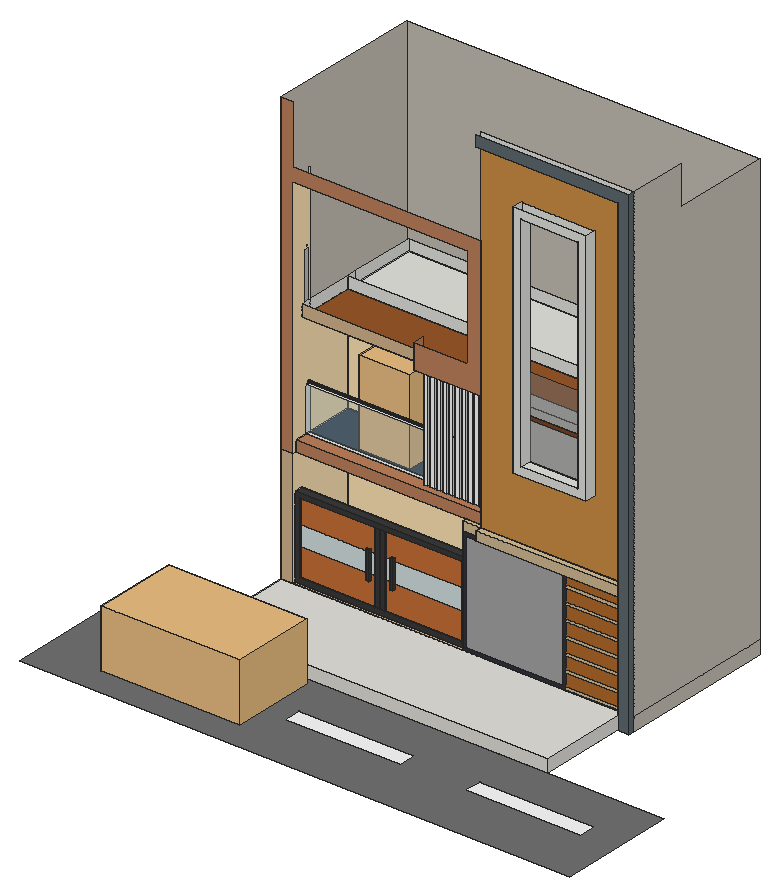
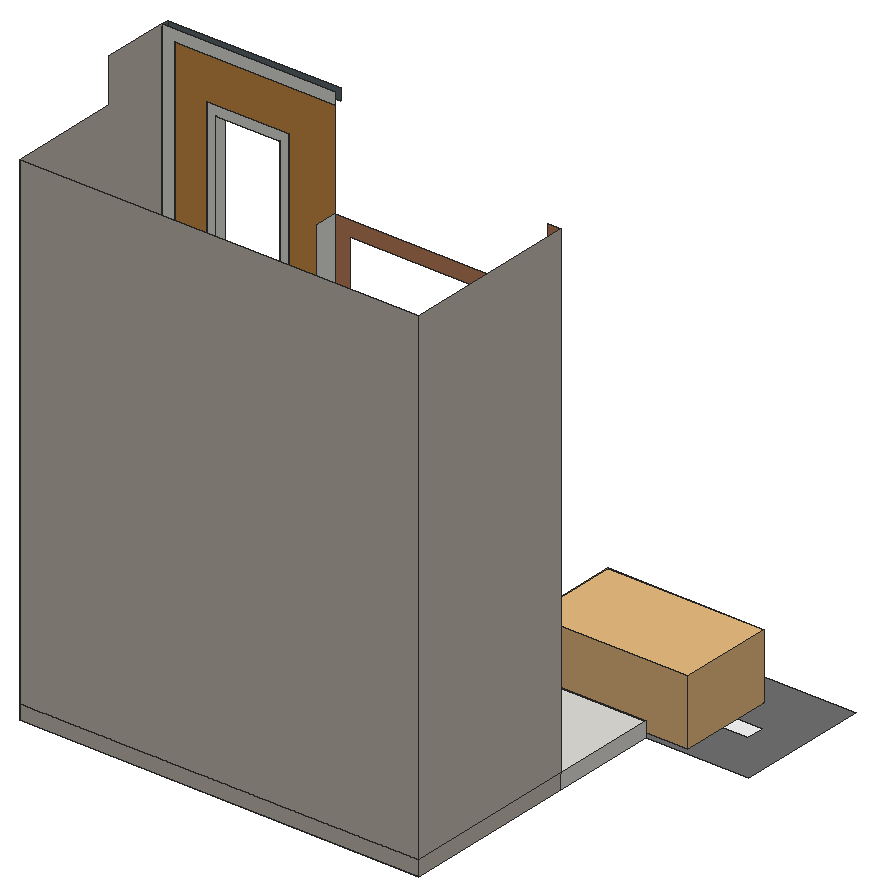
# SketchUp Ruby script. Lengths in inches.
U = 1.inch
M = Sketchup.active_model
def pt(a) = Geom::Point3d.new(a.map { |v| v * U })
def face(e, loops, mat)
  f = e.add_face(loops[0].map { |a| pt(a) })
  loops[1..].each { |l| e.add_face(l.map { |a| pt(a) }).erase! }
  f.material = f.back_material = mat if mat
  f
end
# faces: each face lists its corners as indices into pts; further lists are holes
def faces(e, pts, list, mat = nil) = list.each { |f| face(e, (f[0].is_a?(Array) ? f : [f]).map { |l| l.map { |i| pts[i] } }, mat) }
# xy, xz, yz: faces in a plane at the given z, y or x. An outline is a flat list of corners, or four numbers for a rectangle; further outlines are holes
def ring(l) = l.size == 4 ? [[l[0], l[1]], [l[2], l[1]], [l[2], l[3]], [l[0], l[3]]] : l.each_slice(2).to_a
def flat(e, list, mat, &to3) = list.each { |f| face(e, (f[0].is_a?(Array) ? f : [f]).map { |l| ring(l).map { |u, v| to3.(u, v) } }, mat) }
def xy(e, z, list, mat = nil) = flat(e, list, mat) { |x, y| [x, y, z] }
def xz(e, y, list, mat = nil) = flat(e, list, mat) { |x, z| [x, y, z] }
def yz(e, x, list, mat = nil) = flat(e, list, mat) { |y, z| [x, y, z] }
def lines(e, pts, list) = list.each { |a, b| e.add_line(pt(pts[a]), pt(pts[b])) }
# prism: a flat outline (further loops are holes) pulled along v
def prism(e, loops, v, mat = nil)
  f = face(e, loops, mat); d = Geom::Vector3d.new(v.map { |x| x * U })
  f.pushpull(f.normal.samedirection?(d) ? d.length : -d.length)
end
def box(e, o, s, mat = nil) = prism(e, [[o, [o[0] + s[0], o[1], o[2]], [o[0] + s[0], o[1] + s[1], o[2]], [o[0], o[1] + s[1], o[2]]]], [0, 0, s[2]], mat)
def at(x, y, z, deg = 0) = Geom::Transformation.translation(pt([x, y, z])) * Geom::Transformation.rotation(ORIGIN, Z_AXIS, deg.degrees)
def axes(o, x, y, z) = Geom::Transformation.new([*x, 0, *y, 0, *z, 0, *pt(o).to_a, 1])
def part(name) = M.definitions.add(name)
# library, detail: a bought-in or finely detailed component or shape, given as its bounding box
def library(name, o, s) = part(name).tap { |d| box(d.entities, o, s) }
def detail(e, o, s) = box(e.add_group.entities, o, s)
def put(e, d, t, mat = nil) = e.add_instance(d, t).tap { |i| i.material = mat if mat }
def group(e, t, mat = nil) = e.add_group.tap { |g| g.transformation = t; g.material = mat if mat }.entities
root = M.entities
M.materials.add("[0032_Moccasin]").color = [255, 228, 181]
M.materials.add("[0035_Tan]").color = [210, 180, 140]
M.materials.add("[Carpet Pattern Leaf Squares Tan]").color = [181, 154, 125]
M.materials.add("[Color M05]").color = [114, 114, 114]
M.materials.add("[Color M07]").color = [58, 58, 58]
M.materials.add("[Field Rectangle Tile]").color = [196, 189, 179]
M.materials.add("[Formica Beige]").color = [211, 187, 149]
M.materials.add("[Formica Laminate Dark]").color = [50, 53, 60]
M.materials.add("[Formica Speckled Grey]").color = [94, 105, 111]
M.materials.add("[Leather Blue]").color = [45, 57, 74]
M.materials.add("[Marble Carrara Gold Floor Tile]").color = [225, 223, 217]
M.materials.add("[Quartz Light Grey]").color = [251, 251, 252]
M.materials.add("[Stone Vein Gray]").color = [166, 165, 165]
M.materials.add("[Translucent Glass Gray]").color = [128, 128, 128]
M.materials["[Translucent Glass Gray]"].alpha = 0.5
M.materials.add("[Translucent Glass Safety]").color = [204, 235, 244]
M.materials["[Translucent Glass Safety]"].alpha = 0.14
M.materials.add("[Wallpaper Dog Bone]").color = [213, 224, 224]
M.materials.add("[Wallpaper Stripe]").color = [204, 141, 68]
M.materials.add("[Wood Bamboo]").color = [177, 105, 43]
M.materials.add("[Wood Cherry Original]").color = [198, 112, 54]
M.materials.add("[Wood Cherry Original]1").color = [152, 86, 42]
M.materials.add("[Wood Veneer 01]").color = [120, 70, 37]
M.materials.add("[Wood Veneer 02]").color = [190, 128, 91]
c1 = library("skpE847",[-111.76,-15.01,0.76],[2.12,4.6,1.82])
c2 = part("car+1")
p = [[0,0,0],[1,0,0],[1,1,0]]
lines(c2.entities,p,[[0,1],[1,2],[2,0]])
put(c2.entities,c1,axes([-477.97,5140.8,-31.25],[0,46,0],[-46,0,0],[0,0,40.94]))
c3 = library("chau cay",[-24.34,-109.24,0],[56.46,62.58,79.69])
xy(root,0,[[663.13,313.84,680.56,323.28],[140.56,323.28,680.56,563.28]])
xy(root,0,[[[0,0,841.5625,179.6875],[54.75,86.11,232.01,113.17],[336.5,86.11,513.76,113.17],[612.25,86.11,789.51,113.17]]],"[Color M05]")
xy(root,0,[[140.56,179.6875,663.13,323.28]],"[Marble Carrara Gold Floor Tile]")
xy(root,0,[[54.75,86.11,232.01,113.17],[336.5,86.11,513.76,113.17],[612.25,86.11,789.51,113.17]],"[Quartz Light Grey]")
xy(root,19.8125,[[419.17,323.28,663.13,340.7],[663.13,323.28,680.56,428.92],[157.98,328.46,419.17,340.7],[157.98,428.92,663.13,443.28],[157.98,443.28,663.13,545.86]])
xy(root,19.8125,[[157.98,323.28,419.17,328.46]],"[0035_Tan]")
xy(root,19.8125,[[157.98,340.7,663.13,428.92]],"[Carpet Pattern Leaf Squares Tan]")
xy(root,19.8125,[[140.56,179.6875,663.13,323.28]],"[Marble Carrara Gold Floor Tile]")
xy(root,26.9375,[[279.78,328.46,287.125,340.7],[287.125,328.46,294.47,340.7],[164.55,331.13,279.78,337.5625],[294.47,331.13,413.13,337.5625],[164.55,337.5625,279.78,340.7],
  [294.47,337.5625,413.13,340.7]])
xy(root,26.9375,[[164.55,328.46,279.78,331.13],[294.47,328.46,413.13,331.13]],"[Color M07]")
xy(root,60.02,[[266.23,327.51,271.6,331.13]],"[Color M07]")
xy(root,60.04,[[303.54,327.51,308.36,331.13]],"[Color M07]")
xy(root,103.45,[[266.23,327.51,271.6,331.13]],"[Color M07]")
xy(root,104.22,[[303.54,327.51,308.36,331.13]],"[Color M07]")
xy(root,137.32,[[164.55,328.46,279.78,331.13],[287.125,328.46,294.47,340.7],[294.47,328.46,413.13,331.13],[164.55,331.13,279.78,337.5625],[294.47,331.13,413.13,337.5625],
  [164.55,337.5625,279.78,340.7],[294.47,337.5625,413.13,340.7]])
xy(root,144.0625,[[157.98,328.46,413.13,340.7],[413.13,328.46,419.17,340.7]],"[Color M07]")
xy(root,183.25,[[446.37,313.84,663.13,323.28]],"[Formica Beige]")
xy(root,197.5,[[419.17,329.64,446.37,340.7],[157.98,428.92,663.13,443.28],[157.98,443.28,663.13,545.86]])
xy(root,197.5,[[157.98,329.64,157.98,428.92,663.13,428.92,663.13,340.7,419.17,340.7,419.17,329.64]],"[0035_Tan]")
xy(root,197.5,[[446.37,313.84,663.13,323.28],[419.17,323.28,446.37,329.64]],"[Formica Beige]")
xy(root,213.375,[[345.05,340.7,351.89,346.46],[354.87,340.7,361.71,346.46],[364.24,340.7,371.08,346.46],[373.62,340.7,380.46,346.46],[382.93,340.7,389.77,346.46],
  [393.05,340.7,399.89,346.46],[402.68,340.7,409.52,346.46],[412.87,340.7,419.71,346.46],[422.3,340.7,429.14,346.46],[431.49,340.7,438.33,346.46],
  [440.57,340.7,445.07,346.46],[446.37,340.7,663.13,356.33],[157.98,349.22,446.37,356.33],[157.98,428.92,663.13,443.28],[157.98,443.28,663.13,545.86]])
xy(root,213.375,[[157.98,356.33,663.13,428.92]],"[Leather Blue]")
xy(root,213.375,[[[157.98,329.64,446.37,349.22],[393.05,340.7,399.89,346.46],[402.68,340.7,409.52,346.46],[354.87,340.7,361.71,346.46],[364.24,340.7,371.08,346.46],[345.05,340.7,351.89,346.46],[382.93,340.7,389.77,346.46],[373.62,340.7,380.46,346.46],[422.3,340.7,429.14,346.46],[412.87,340.7,419.71,346.46],[431.49,340.7,438.33,346.46],[440.57,340.7,445.07,346.46]]],"[Wood Veneer 02]")
xy(root,281.5625,[[157.98,349.22,446.37,356.33]])
xy(root,301.64,[[508.84,307.03,620.21,323.28]])
xy(root,314.02,[[521.21,307.03,607.83,323.28]])
xy(root,377.5,[[345.05,340.7,351.89,346.46],[446.37,340.7,663.13,356.33],[157.98,428.92,663.13,443.28],[157.98,443.28,663.13,545.86]])
xy(root,377.5,[[157.98,340.7,157.98,428.92,663.13,428.92,663.13,356.33,446.37,356.33,446.37,340.7,445.07,340.7,445.07,346.46,440.57,346.46,440.57,340.7,438.33,340.7,438.33,346.46,431.49,346.46,431.49,340.7,429.14,340.7,429.14,346.46,422.3,346.46,422.3,340.7,419.71,340.7,419.71,346.46,412.87,346.46,412.87,340.7,409.52,340.7,409.52,346.46,402.68,346.46,402.68,340.7,399.89,340.7,399.89,346.46,393.05,346.46,393.05,340.7,389.77,340.7,389.77,346.46,382.93,346.46,382.93,340.7,380.46,340.7,380.46,346.46,373.62,346.46,373.62,340.7,371.08,340.7,371.08,346.46,364.24,346.46,364.24,340.7,361.71,340.7,361.71,346.46,354.87,346.46,354.87,340.7,351.89,340.7,351.89,346.46,345.05,346.46,345.05,340.7]],"[Wood Cherry Original]1")
xy(root,377.5,[[343.27,323.28,446.37,340.7]],"[Wood Veneer 02]")
xz(root,179.6875,[[140.56,0,663.13,19.8125]],"[Marble Carrara Gold Floor Tile]")
xz(root,307.03,[[[508.84,301.64,620.21,665.95],[521.21,314.02,607.83,653.58]]])
xz(root,313.84,[[446.37,183.25,663.13,197.5]],"[Formica Beige]")
xz(root,313.84,[[663.13,0,680.56,0,680.56,739.5,446.37,739.5,446.37,723.61,663.13,723.61]],"[Formica Speckled Grey]")
xz(root,323.28,[[663.13,0,680.56,19.8125],[663.13,19.8125,663.13,723.61,446.37,723.61,446.37,739.5,680.56,739.5,680.56,19.8125],[446.37,183.25,663.13,197.5],[[508.84,301.64,620.21,665.95],[521.21,314.02,607.83,653.58]]])
xz(root,323.28,[[140.56,19.8125,157.98,197.5]],"[0035_Tan]")
xz(root,323.28,[[577.04,19.8125,663.13,20.9375],[577.04,20.9375,663.13,25.12],[577.04,44.125,663.13,48.31],[577.04,67.3125,663.13,71.5],[577.04,90.5,663.13,94.68],
  [577.04,113.6875,663.13,117.87],[577.04,136.875,663.13,141.06],[577.04,160.0625,663.13,164.25],[419.17,183.25,446.37,197.5]],"[Formica Beige]")
xz(root,323.28,[[[419.17,19.8125,577.04,183.25],[423.9,24.55,572.3125,178.52]]],"[Formica Laminate Dark]")
xz(root,323.28,[[140.56,0,577.04,19.8125],[577.04,0,663.13,1.93]],"[Marble Carrara Gold Floor Tile]")
xz(root,323.28,[[423.9,24.55,572.3125,178.52]],"[Stone Vein Gray]")
xz(root,323.28,[[521.21,314.02,607.83,371.81],[521.21,377.6,607.83,437.62]],"[Translucent Glass Gray]")
xz(root,323.28,[[[446.37,197.5,663.13,723.61],[508.84,301.64,620.21,665.95]]],"[Wallpaper Stripe]")
xz(root,323.28,[[577.04,1.93,663.13,19.8125],[577.04,25.12,663.13,44.125],[577.04,48.31,663.13,67.3125],[577.04,71.5,663.13,90.5],[577.04,94.68,663.13,113.6875],
  [577.04,117.87,663.13,136.875],[577.04,141.06,663.13,160.0625],[577.04,164.25,663.13,183.25]],"[Wood Bamboo]")
xz(root,323.28,[[521.21,371.81,607.83,377.6]],"[Wood Veneer 01]")
xz(root,323.28,[[140.56,197.5,157.98,197.5,157.98,570.15,426.08,570.15,426.08,414.6875,343.27,414.6875,343.27,377.5,446.37,377.5,446.37,590.9375,157.98,590.9375,157.98,680.125,140.56,680.125]],"[Wood Veneer 02]")
xz(root,327.51,[[266.23,60.02,271.6,103.45],[303.54,60.04,308.36,104.22]],"[Color M07]")
xz(root,328.46,[[[157.98,19.8125,419.17,144.0625],[164.55,26.9375,413.13,137.32]],[279.78,26.9375,287.125,137.32],[287.125,26.9375,294.47,137.32]],"[Color M07]")
xz(root,329.64,[[157.98,197.5,446.37,213.375]],"[Wood Veneer 02]")
xz(root,331.13,[[266.23,60.02,271.6,103.45],[303.54,60.04,308.36,104.22]],"[Color M07]")
xz(root,331.13,[[294.47,68.5,303.54,99.11],[308.36,68.5,413.13,99.11],[164.55,68.81,266.23,99.32],[271.6,68.81,279.78,99.32]],"[Wallpaper Dog Bone]")
xz(root,331.13,[[164.55,26.9375,279.78,26.9375,279.78,68.81,271.6,68.81,271.6,60.02,266.23,60.02,266.23,68.81,164.55,68.81],[294.47,26.9375,413.13,26.9375,413.13,68.5,308.36,68.5,308.36,60.04,303.54,60.04,303.54,68.5,294.47,68.5],[294.47,99.11,303.54,99.11,303.54,104.22,308.36,104.22,308.36,99.11,413.13,99.11,413.13,137.32,294.47,137.32],[164.55,99.32,266.23,99.32,266.23,103.45,271.6,103.45,271.6,99.32,279.78,99.32,279.78,137.32,164.55,137.32]],"[Wood Cherry Original]")
xz(root,337.5625,[[164.55,26.9375,279.78,137.32],[294.47,26.9375,413.13,137.32]])
xz(root,340.7,[[[157.98,19.8125,419.17,144.0625],[164.55,26.9375,413.13,137.32]],[279.78,26.9375,287.125,137.32],[287.125,26.9375,294.47,137.32],[446.37,197.5,663.13,213.375],[343.27,377.5,446.37,394.8125],
  [446.37,377.5,663.13,394.8125]])
xz(root,340.7,[[157.98,377.5,343.27,394.8125]],"[0035_Tan]")
xz(root,340.7,[[419.17,19.8125,663.13,197.5]],"[Formica Beige]")
xz(root,340.7,[[345.05,213.375,351.89,377.5],[354.87,213.375,361.71,377.5],[364.24,213.375,371.08,377.5],[373.62,213.375,380.46,377.5],[382.93,213.375,389.77,377.5],
  [393.05,213.375,399.89,377.5],[402.68,213.375,409.52,377.5],[412.87,213.375,419.71,377.5],[422.3,213.375,429.14,377.5],[431.49,213.375,438.33,377.5],
  [440.57,213.375,445.07,377.5]],"[Quartz Light Grey]")
xz(root,346.46,[[345.05,213.375,351.89,377.5],[354.87,213.375,361.71,377.5],[364.24,213.375,371.08,377.5],[373.62,213.375,380.46,377.5],[382.93,213.375,389.77,377.5],
  [393.05,213.375,399.89,377.5],[402.68,213.375,409.52,377.5],[412.87,213.375,419.71,377.5],[422.3,213.375,429.14,377.5],[431.49,213.375,438.33,377.5],
  [440.57,213.375,445.07,377.5]])
xz(root,349.22,[[157.98,213.375,446.37,281.5625]],"[Translucent Glass Safety]")
xz(root,356.33,[[446.37,213.375,663.13,377.5]])
xz(root,356.33,[[157.98,213.375,446.37,281.5625]],"[Translucent Glass Safety]")
xz(root,428.92,[[157.98,197.5,663.13,213.375],[157.98,377.5,663.13,394.8125]])
xz(root,428.92,[[157.98,19.8125,663.13,197.5],[157.98,213.375,663.13,377.5]],"[0032_Moccasin]")
xz(root,443.28,[[157.98,19.8125,663.13,197.5],[157.98,197.5,663.13,213.375],[157.98,213.375,663.13,377.5]])
xz(root,545.86,[[157.98,19.8125,663.13,197.5],[157.98,197.5,663.13,213.375],[157.98,213.375,663.13,377.5],[157.98,377.5,663.13,394.8125]])
xz(root,563.28,[[140.56,0,680.56,19.8125],[140.56,19.8125,680.56,680.125]],"[Field Rectangle Tile]")
yz(root,140.56,[[323.28,0,563.28,19.8125],[323.28,19.8125,563.28,680.125]],"[Field Rectangle Tile]")
yz(root,140.56,[[179.6875,0,323.28,19.8125]],"[Marble Carrara Gold Floor Tile]")
yz(root,157.98,[[328.46,19.8125,340.7,144.0625],[428.92,19.8125,443.28,197.5],[443.28,19.8125,545.86,197.5],[329.64,197.5,428.92,213.375],[428.92,197.5,443.28,213.375],
  [443.28,197.5,545.86,213.375],[349.22,213.375,356.33,281.5625],[428.92,213.375,443.28,377.5],[443.28,213.375,545.86,377.5],[352.3125,283.62,351.97,283.66,351.66,283.79,351.39,284,351.18,284.27,351.05,284.59,351,284.93,351.05,285.27,351.18,285.58,351.39,285.86,351.66,286.06,351.97,286.2,352.3125,286.24,352.65,286.2,352.97,286.06,353.24,285.86,353.45,285.58,353.58,285.27,353.625,284.93,353.58,284.59,353.45,284.27,353.24,284,352.97,283.79,352.65,283.66],
  [340.7,377.5,356.33,394.8125],[356.33,377.5,428.92,394.8125],[428.92,377.5,443.28,394.8125],[443.28,377.5,545.86,394.8125]])
yz(root,157.98,[[323.28,19.8125,328.46,19.8125,328.46,144.0625,340.7,144.0625,340.7,19.8125,428.92,19.8125,428.92,197.5,323.28,197.5],[[323.28,197.5,329.64,197.5,329.64,213.375,349.22,213.375,349.22,281.5625,356.33,281.5625,356.33,213.375,428.92,213.375,428.92,377.5,340.7,377.5,340.7,394.8125,345.57,394.8125,345.57,467.1875,354.64,467.1875,354.64,394.8125,356.33,394.8125,356.33,576.33,354.64,576.33,354.64,570.15,323.28,570.15],[350.17,469.16,349.6,469.23,349.07,469.45,348.62,469.8,348.27,470.25,348.05,470.78,347.98,471.34,348.05,471.91,348.27,472.4375,348.62,472.89,349.07,473.24,349.6,473.46,350.17,473.53,350.73,473.46,351.26,473.24,351.71,472.89,352.06,472.4375,352.28,471.91,352.35,471.34,352.28,470.78,352.06,470.25,351.71,469.8,351.26,469.45,350.73,469.23],[352.3125,283.62,351.97,283.66,351.66,283.79,351.39,284,351.18,284.27,351.05,284.59,351,284.93,351.05,285.27,351.18,285.58,351.39,285.86,351.66,286.06,351.97,286.2,352.3125,286.24,352.65,286.2,352.97,286.06,353.24,285.86,353.45,285.58,353.58,285.27,353.625,284.93,353.58,284.59,353.45,284.27,353.24,284,352.97,283.79,352.65,283.66]]],"[0032_Moccasin]")
yz(root,164.55,[[331.13,26.9375,337.5625,137.32],[337.5625,26.9375,340.7,137.32]])
yz(root,164.55,[[328.46,26.9375,331.13,137.32]],"[Color M07]")
yz(root,266.23,[[327.51,60.02,331.13,68.81],[327.51,68.81,331.13,99.32],[327.51,99.32,331.13,103.45]],"[Color M07]")
yz(root,271.6,[[327.51,60.02,331.13,68.81],[327.51,68.81,331.13,99.32],[327.51,99.32,331.13,103.45]],"[Color M07]")
yz(root,279.78,[[331.13,26.9375,337.5625,137.32],[337.5625,26.9375,340.7,137.32]])
yz(root,279.78,[[328.46,26.9375,331.13,137.32]],"[Color M07]")
yz(root,287.125,[[328.46,26.9375,340.7,137.32]])
yz(root,294.47,[[331.13,26.9375,337.5625,137.32],[337.5625,26.9375,340.7,137.32]])
yz(root,294.47,[[328.46,26.9375,331.13,137.32]],"[Color M07]")
yz(root,303.54,[[327.51,60.04,331.13,68.5],[327.51,68.5,331.13,99.11],[327.51,99.11,331.13,104.22]],"[Color M07]")
yz(root,308.36,[[327.51,60.04,331.13,68.5],[327.51,68.5,331.13,99.11],[327.51,99.11,331.13,104.22]],"[Color M07]")
yz(root,343.27,[[323.28,377.5,340.7,414.6875]],"[Wood Veneer 02]")
yz(root,345.05,[[340.7,213.375,346.46,377.5]],"[Quartz Light Grey]")
yz(root,351.89,[[340.7,213.375,346.46,377.5]])
yz(root,354.87,[[340.7,213.375,346.46,377.5]],"[Quartz Light Grey]")
yz(root,361.71,[[340.7,213.375,346.46,377.5]])
yz(root,364.24,[[340.7,213.375,346.46,377.5]],"[Quartz Light Grey]")
yz(root,371.08,[[340.7,213.375,346.46,377.5]])
yz(root,373.62,[[340.7,213.375,346.46,377.5]],"[Quartz Light Grey]")
yz(root,380.46,[[340.7,213.375,346.46,377.5]])
yz(root,382.93,[[340.7,213.375,346.46,377.5]],"[Quartz Light Grey]")
yz(root,389.77,[[340.7,213.375,346.46,377.5]])
yz(root,393.05,[[340.7,213.375,346.46,377.5]],"[Quartz Light Grey]")
yz(root,399.89,[[340.7,213.375,346.46,377.5]])
yz(root,402.68,[[340.7,213.375,346.46,377.5]],"[Quartz Light Grey]")
yz(root,409.52,[[340.7,213.375,346.46,377.5]])
yz(root,412.87,[[340.7,213.375,346.46,377.5]],"[Quartz Light Grey]")
yz(root,413.13,[[331.13,26.9375,337.5625,137.32],[337.5625,26.9375,340.7,137.32]])
yz(root,413.13,[[328.46,26.9375,331.13,137.32]],"[Color M07]")
yz(root,419.17,[[328.46,19.8125,340.7,144.0625]])
yz(root,419.17,[[323.28,19.8125,323.28,197.5,340.7,197.5,340.7,144.0625,328.46,144.0625,328.46,19.8125]],"[Formica Beige]")
yz(root,419.71,[[340.7,213.375,346.46,377.5]])
yz(root,422.3,[[340.7,213.375,346.46,377.5]],"[Quartz Light Grey]")
yz(root,429.14,[[340.7,213.375,346.46,377.5]])
yz(root,431.49,[[340.7,213.375,346.46,377.5]],"[Quartz Light Grey]")
yz(root,438.33,[[340.7,213.375,346.46,377.5]])
yz(root,440.57,[[340.7,213.375,346.46,377.5]],"[Quartz Light Grey]")
yz(root,445.07,[[340.7,213.375,346.46,377.5]])
yz(root,446.37,[[329.64,197.5,340.7,213.375],[323.28,377.5,340.7,377.5,340.7,394.8125,343.6,394.8125,343.6,467.1875,354.64,467.1875,354.64,590.9375,323.28,590.9375]])
yz(root,446.37,[[313.84,183.25,323.28,197.5]],"[Formica Beige]")
yz(root,446.37,[[[323.28,197.5,323.28,377.5,356.33,377.5,356.33,281.5625,349.22,281.5625,349.22,213.375,329.64,213.375,329.64,197.5],[352.3125,283.62,352.65,283.66,352.97,283.79,353.24,284,353.45,284.27,353.58,284.59,353.625,284.93,353.58,285.27,353.45,285.58,353.24,285.86,352.97,286.06,352.65,286.2,352.3125,286.24,351.97,286.2,351.66,286.06,351.39,285.86,351.18,285.58,351.05,285.27,351,284.93,351.05,284.59,351.18,284.27,351.39,284,351.66,283.79,351.97,283.66]]],"[Wood Cherry Original]1")
yz(root,508.84,[[307.03,301.64,323.28,665.95]])
yz(root,521.21,[[307.03,314.02,323.28,653.58]])
yz(root,607.83,[[307.03,314.02,323.28,653.58]])
yz(root,620.21,[[307.03,301.64,323.28,665.95]])
yz(root,663.13,[[428.92,19.8125,443.28,197.5],[443.28,19.8125,545.86,197.5],[313.84,183.25,323.28,197.5],[340.7,197.5,428.92,213.375],[428.92,197.5,443.28,213.375],
  [443.28,197.5,545.86,213.375],[428.92,213.375,443.28,377.5],[443.28,213.375,545.86,377.5],[340.7,377.5,356.33,394.8125],[356.33,377.5,428.92,394.8125],
  [428.92,377.5,443.28,394.8125],[443.28,377.5,545.86,394.8125]])
yz(root,663.13,[[340.7,19.8125,428.92,197.5],[356.33,213.375,428.92,377.5]],"[0032_Moccasin]")
yz(root,663.13,[[313.84,19.8125,323.28,183.25],[313.84,197.5,323.28,723.61]],"[Formica Speckled Grey]")
yz(root,663.13,[[179.6875,0,313.84,19.8125],[313.84,0,323.28,19.8125]],"[Marble Carrara Gold Floor Tile]")
yz(root,680.56,[[323.28,0,563.28,19.8125],[323.28,19.8125,563.28,19.8125,563.28,680.125,412.7,680.125,412.7,739.5,323.28,739.5]],"[Field Rectangle Tile]")
yz(root,680.56,[[313.84,0,323.28,739.5]],"[Formica Speckled Grey]")
p = [[157.98,351.97,283.66],[157.98,352.3125,283.62],[446.37,352.3125,283.62],[446.37,351.97,283.66],[157.98,352.65,283.66],[446.37,352.65,283.66],
  [157.98,351.66,283.79],[446.37,351.66,283.79],[157.98,352.97,283.79],[446.37,352.97,283.79],[157.98,351.39,284],[446.37,351.39,284],
  [157.98,353.24,284],[446.37,353.24,284],[157.98,351.18,284.27],[446.37,351.18,284.27],[157.98,353.45,284.27],[446.37,353.45,284.27],
  [157.98,351.05,284.59],[446.37,351.05,284.59],[157.98,353.58,284.59],[446.37,353.58,284.59],[157.98,351,284.93],[446.37,351,284.93],
  [157.98,353.625,284.93],[446.37,353.625,284.93],[157.98,351.05,285.27],[446.37,351.05,285.27],[157.98,353.58,285.27],[446.37,353.58,285.27],
  [157.98,351.18,285.58],[446.37,351.18,285.58],[157.98,353.45,285.58],[446.37,353.45,285.58],[157.98,351.39,285.86],[446.37,351.39,285.86],
  [157.98,353.24,285.86],[446.37,353.24,285.86],[157.98,351.66,286.06],[446.37,351.66,286.06],[157.98,352.97,286.06],[446.37,352.97,286.06],
  [157.98,351.97,286.2],[446.37,351.97,286.2],[157.98,352.65,286.2],[446.37,352.65,286.2],[157.98,352.3125,286.24],[446.37,352.3125,286.24]]
faces(root,p,[[0,1,2,3],[1,4,5,2],[6,0,3,7],[4,8,9,5],[10,6,7,11],[8,12,13,9],[14,10,11,15],[12,16,17,13],
  [18,14,15,19],[16,20,21,17],[22,18,19,23],[20,24,25,21],[26,22,23,27],[24,28,29,25],[30,26,27,31],[28,32,33,29],
  [34,30,31,35],[32,36,37,33],[38,34,35,39],[36,40,41,37],[42,38,39,43],[40,44,45,41],[46,42,43,47],[44,46,47,45]],"[Color M07]")
put(root,c2,axes([89.34,42.39,0],[1,0,0],[0,1.3224,0],[0,0,1.19]))
put(root,c3,axes([264.13,469.24,213.375],[1.3699,0,0],[0,1,0],[0,0,1.6146]))
